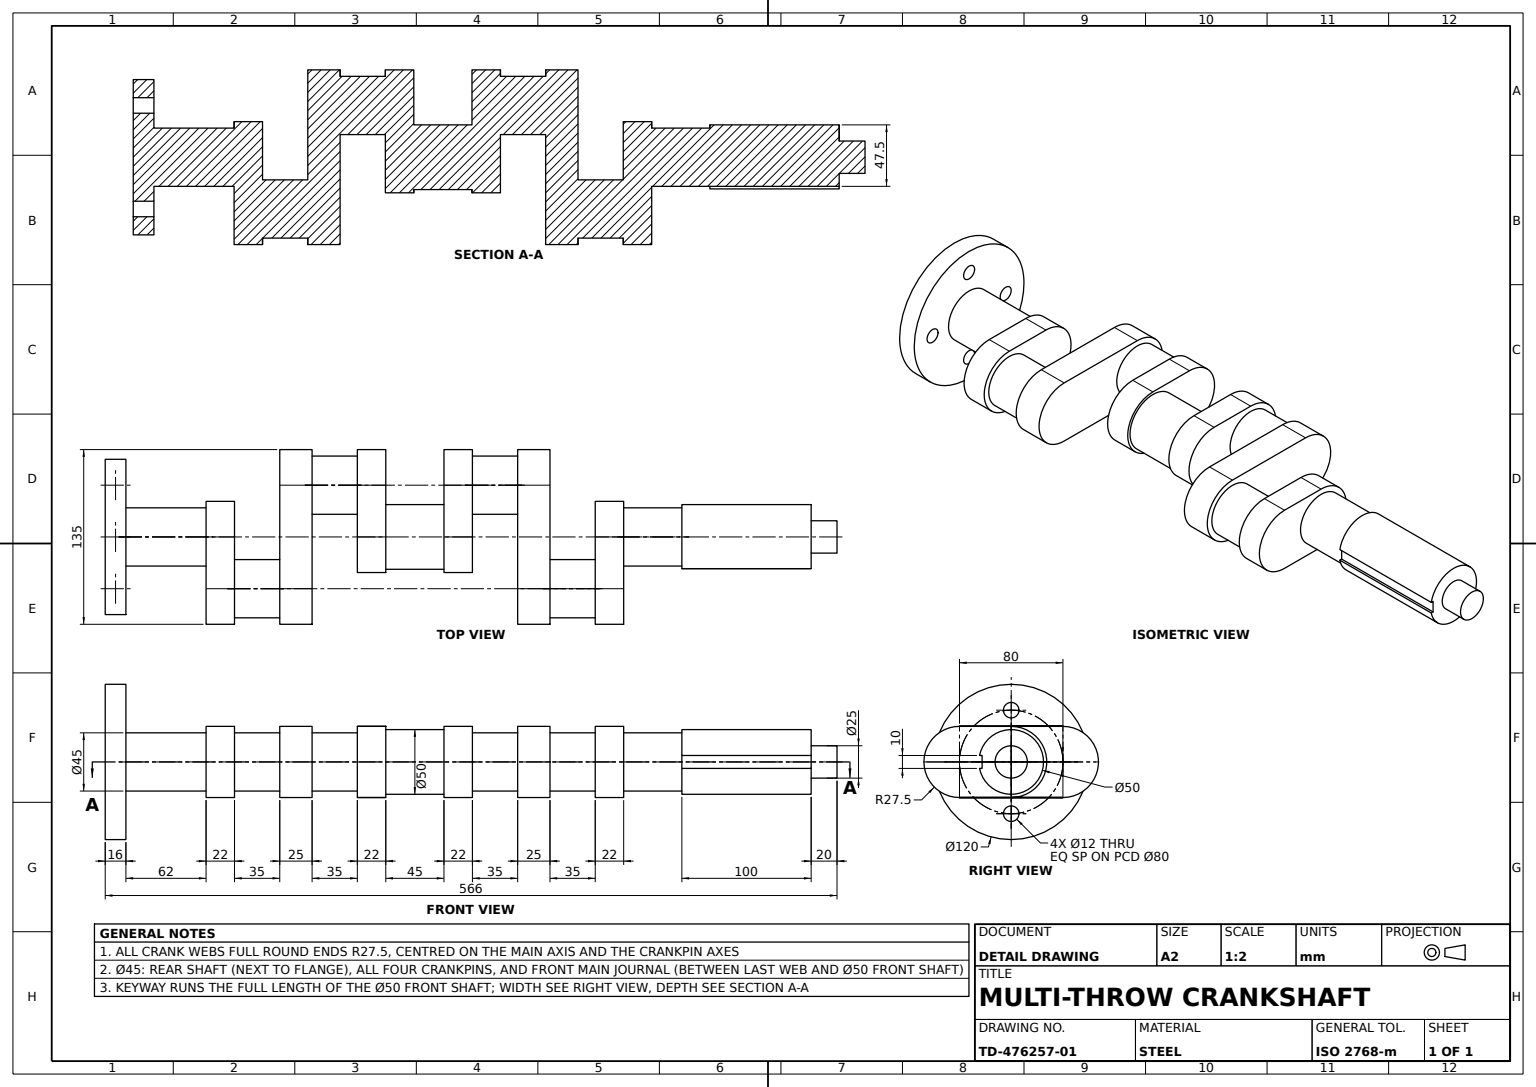
solid
v1 (262,-27.5,0)
v2 (262,-27.5,-40)
e1 v1 v2 LINE
v3 (262,0,27.5)
e2 v3 v1 CIRCLE(AX(P(262,0,0),D(1,0,0),D(0,0,-1)),27.5)
v4 (262,27.5,0)
e3 v4 v3 CIRCLE(AX(P(262,0,0),D(1,0,0),D(0,0,-1)),27.5)
v5 (262,27.5,-40)
e4 v5 v4 LINE
e5 v2 v5 CIRCLE(AX(P(262,0,-40),D(1,0,0),D(0,0,-1)),27.5)
v6 (262,0,25)
v7 (262,0,-25)
e6 v6 v7 CIRCLE(AX(P(262,0,0),D(1,0,0),D(0,0,-1)),25)
e7 v7 v6 CIRCLE(AX(P(262,0,0),D(1,0,0),D(0,0,-1)),25)
face PLANE(AX(P(262,0,0),D(1,0,0),D(0,0,-1))) rev [-e1 -e2 -e3 -e4 -e5] [e6 e7]
v8 (78,0,-22.5)
v9 (78,0,22.5)
e8 v8 v9 CIRCLE(AX(P(78,0,0),D(-1,0,0),D(0,0,1)),22.5)
e9 v9 v8 CIRCLE(AX(P(78,0,0),D(-1,0,0),D(0,0,1)),22.5)
v10 (78,0,67.5)
v11 (78,-27.5,40)
e10 v10 v11 CIRCLE(AX(P(78,0,40),D(1,0,0),D(0,0,-1)),27.5)
v12 (78,27.5,40)
e11 v12 v10 CIRCLE(AX(P(78,0,40),D(1,0,0),D(0,0,-1)),27.5)
v13 (78,27.5,0)
e12 v13 v12 LINE
v14 (78,-27.5,0)
e13 v14 v13 CIRCLE(AX(P(78,0,0),D(1,0,0),D(0,0,-1)),27.5)
e14 v11 v14 LINE
face PLANE(AX(P(78,0,0),D(1,0,0),D(0,0,-1))) rev [-e8 -e9] [-e10 -e11 -e12 -e13 -e14]
v15 (16,-40,6)
v16 (0,-40,6)
e15 v15 v16 LINE
v17 (16,-40,-6)
e16 v17 v15 CIRCLE(AX(P(16,-40,0),D(-1,0,0),D(0,0,1)),6)
v18 (0,-40,-6)
e17 v17 v18 LINE
e18 v18 v16 CIRCLE(AX(P(0,-40,0),D(-1,0,0),D(0,0,1)),6)
face CYL(AX(P(20,-40,0),D(-1,0,0),D(0,0,1)),6) rev [-e15 -e16 e17 e18]
v19 (160,-27.5,-40)
v20 (160,27.5,-40)
e19 v19 v20 CIRCLE(AX(P(160,0,-40),D(1,0,0),D(0,0,-1)),27.5)
v21 (160,27.5,40)
e20 v20 v21 LINE
v22 (160,0,67.5)
e21 v21 v22 CIRCLE(AX(P(160,0,40),D(1,0,0),D(0,0,-1)),27.5)
v23 (160,-27.5,40)
e22 v22 v23 CIRCLE(AX(P(160,0,40),D(1,0,0),D(0,0,-1)),27.5)
e23 v23 v19 LINE
v24 (160,0,-62.5)
v25 (160,0,-17.5)
e24 v24 v25 CIRCLE(AX(P(160,0,-40),D(1,0,0),D(0,0,-1)),22.5)
e25 v25 v24 CIRCLE(AX(P(160,0,-40),D(1,0,0),D(0,0,-1)),22.5)
face PLANE(AX(P(160,0,40),D(1,0,0),D(0,0,-1))) [e19 e20 e21 e22 e23] [-e24 -e25]
v26 (284,27.5,-40)
e26 v26 v5 LINE
v27 (284,27.5,0)
e27 v27 v4 LINE
e28 v26 v27 LINE
face PLANE(AX(P(284,27.5,0),D(0,-1,0),D(0,0,-1))) rev [e26 e4 -e27 -e28]
v28 (319,0,-62.5)
v29 (319,0,-17.5)
e29 v28 v29 CIRCLE(AX(P(319,0,-40),D(1,0,0),D(0,0,-1)),22.5)
e30 v29 v28 CIRCLE(AX(P(319,0,-40),D(1,0,0),D(0,0,-1)),22.5)
v30 (319,27.5,40)
v31 (319,0,67.5)
e31 v30 v31 CIRCLE(AX(P(319,0,40),D(1,0,0),D(0,0,-1)),27.5)
v32 (319,27.5,-40)
e32 v32 v30 LINE
v33 (319,-27.5,-40)
e33 v33 v32 CIRCLE(AX(P(319,0,-40),D(1,0,0),D(0,0,-1)),27.5)
v34 (319,-27.5,40)
e34 v34 v33 LINE
e35 v31 v34 CIRCLE(AX(P(319,0,40),D(1,0,0),D(0,0,-1)),27.5)
face PLANE(AX(P(319,0,-40),D(1,0,0),D(0,0,-1))) rev [e29 e30] [-e31 -e32 -e33 -e34 -e35]
v35 (217,27.5,-40)
v36 (217,27.5,0)
e36 v35 v36 LINE
v37 (217,0,27.5)
e37 v36 v37 CIRCLE(AX(P(217,0,0),D(1,0,0),D(0,0,-1)),27.5)
v38 (217,-27.5,0)
e38 v37 v38 CIRCLE(AX(P(217,0,0),D(1,0,0),D(0,0,-1)),27.5)
v39 (217,-27.5,-40)
e39 v38 v39 LINE
e40 v39 v35 CIRCLE(AX(P(217,0,-40),D(1,0,0),D(0,0,-1)),27.5)
v40 (217,0,25)
v41 (217,0,-25)
e41 v40 v41 CIRCLE(AX(P(217,0,0),D(1,0,0),D(0,0,-1)),25)
e42 v41 v40 CIRCLE(AX(P(217,0,0),D(1,0,0),D(0,0,-1)),25)
face PLANE(AX(P(217,0,-40),D(1,0,0),D(0,0,-1))) [e36 e37 e38 e39 e40] [-e41 -e42]
v42 (401,27.5,40)
v43 (401,0,67.5)
e43 v42 v43 CIRCLE(AX(P(401,0,40),D(1,0,0),D(0,0,-1)),27.5)
v44 (379,27.5,40)
e44 v42 v44 LINE
v45 (379,0,67.5)
e45 v44 v45 CIRCLE(AX(P(379,0,40),D(1,0,0),D(0,0,-1)),27.5)
e46 v43 v45 LINE
face CYL(AX(P(401,0,40),D(-1,0,0),D(0,0,1)),27.5) [-e43 e44 e45 -e46]
v46 (0,0,-34)
v47 (0,0,-46)
e47 v46 v47 CIRCLE(AX(P(0,0,-40),D(-1,0,0),D(0,0,1)),6)
v48 (16,0,-46)
e48 v48 v47 LINE
v49 (16,0,-34)
e49 v49 v48 CIRCLE(AX(P(16,0,-40),D(-1,0,0),D(0,0,1)),6)
e50 v49 v46 LINE
face CYL(AX(P(20,0,-40),D(-1,0,0),D(0,0,1)),6) rev [e47 -e48 -e49 e50]
v50 (446,5,22.5)
v51 (546,5,22.5)
e51 v50 v51 LINE
v52 (446,0,22.5)
e52 v52 v50 LINE
v53 (446,-5,22.5)
e53 v53 v52 LINE
v54 (546,-5,22.5)
e54 v53 v54 LINE
e55 v54 v51 LINE
face PLANE(AX(P(436,5,22.5),D(0,0,-1),D(-1,0,0))) rev [-e51 -e52 -e53 e54 e55]
v55 (566,0,12.5)
v56 (546,0,12.5)
e56 v55 v56 LINE
v57 (566,0,-12.5)
e57 v57 v55 CIRCLE(AX(P(566,0,0),D(1,0,0),D(0,0,-1)),12.5)
v58 (546,0,-12.5)
e58 v57 v58 LINE
e59 v58 v56 CIRCLE(AX(P(546,0,0),D(1,0,0),D(0,0,-1)),12.5)
face CYL(AX(P(566,0,0),D(-1,0,0),D(0,0,1)),12.5) [-e56 -e57 e58 e59]
e60 v15 v17 CIRCLE(AX(P(16,-40,0),D(-1,0,0),D(0,0,1)),6)
e61 v16 v18 CIRCLE(AX(P(0,-40,0),D(-1,0,0),D(0,0,1)),6)
face CYL(AX(P(20,-40,0),D(-1,0,0),D(0,0,1)),6) rev [-e60 e15 e61 -e17]
v59 (401,-27.5,0)
v60 (401,27.5,0)
e62 v59 v60 CIRCLE(AX(P(401,0,0),D(1,0,0),D(0,0,-1)),27.5)
e63 v60 v42 LINE
v61 (401,-27.5,40)
e64 v43 v61 CIRCLE(AX(P(401,0,40),D(1,0,0),D(0,0,-1)),27.5)
e65 v61 v59 LINE
v62 (401,0,22.5)
v63 (401,0,-22.5)
e66 v62 v63 CIRCLE(AX(P(401,0,0),D(1,0,0),D(0,0,-1)),22.5)
e67 v63 v62 CIRCLE(AX(P(401,0,0),D(1,0,0),D(0,0,-1)),22.5)
face PLANE(AX(P(401,0,40),D(1,0,0),D(0,0,-1))) [e62 e63 e43 e64 e65] [-e66 -e67]
v64 (446,5,24.494897)
v65 (546,5,24.494897)
e68 v64 v65 LINE
e69 v50 v64 LINE
e70 v51 v65 LINE
face PLANE(AX(P(436,5,27.5),D(0,1,0),D(0,0,1))) rev [-e68 -e69 e51 e70]
v66 (284,0,-17.5)
e71 v29 v66 LINE
v67 (284,0,-62.5)
e72 v66 v67 CIRCLE(AX(P(284,0,-40),D(1,0,0),D(0,0,-1)),22.5)
e73 v28 v67 LINE
face CYL(AX(P(319,0,-40),D(-1,0,0),D(0,0,1)),22.5) [e71 e72 -e73 -e30]
v68 (344,0,17.5)
v69 (344,0,62.5)
e74 v68 v69 CIRCLE(AX(P(344,0,40),D(1,0,0),D(0,0,-1)),22.5)
v70 (379,0,62.5)
e75 v70 v69 LINE
v71 (379,0,17.5)
e76 v71 v70 CIRCLE(AX(P(379,0,40),D(1,0,0),D(0,0,-1)),22.5)
e77 v71 v68 LINE
face CYL(AX(P(379,0,40),D(-1,0,0),D(0,0,1)),22.5) [e74 -e75 -e76 e77]
v72 (195,-27.5,0)
v73 (195,-27.5,-40)
e78 v72 v73 LINE
v74 (195,0,27.5)
e79 v74 v72 CIRCLE(AX(P(195,0,0),D(1,0,0),D(0,0,-1)),27.5)
v75 (195,27.5,0)
e80 v75 v74 CIRCLE(AX(P(195,0,0),D(1,0,0),D(0,0,-1)),27.5)
v76 (195,27.5,-40)
e81 v76 v75 LINE
e82 v73 v76 CIRCLE(AX(P(195,0,-40),D(1,0,0),D(0,0,-1)),27.5)
v77 (195,0,-62.5)
v78 (195,0,-17.5)
e83 v77 v78 CIRCLE(AX(P(195,0,-40),D(1,0,0),D(0,0,-1)),22.5)
e84 v78 v77 CIRCLE(AX(P(195,0,-40),D(1,0,0),D(0,0,-1)),22.5)
face PLANE(AX(P(195,0,-40),D(1,0,0),D(0,0,-1))) rev [-e78 -e79 -e80 -e81 -e82] [e83 e84]
v79 (135,0,62.5)
v80 (135,0,17.5)
e85 v79 v80 CIRCLE(AX(P(135,0,40),D(1,0,0),D(0,0,-1)),22.5)
e86 v80 v79 CIRCLE(AX(P(135,0,40),D(1,0,0),D(0,0,-1)),22.5)
v81 (135,-27.5,-40)
v82 (135,27.5,-40)
e87 v81 v82 CIRCLE(AX(P(135,0,-40),D(1,0,0),D(0,0,-1)),27.5)
v83 (135,-27.5,40)
e88 v83 v81 LINE
v84 (135,0,67.5)
e89 v84 v83 CIRCLE(AX(P(135,0,40),D(1,0,0),D(0,0,-1)),27.5)
v85 (135,27.5,40)
e90 v85 v84 CIRCLE(AX(P(135,0,40),D(1,0,0),D(0,0,-1)),27.5)
e91 v82 v85 LINE
face PLANE(AX(P(135,0,40),D(1,0,0),D(0,0,-1))) rev [e85 e86] [-e87 -e88 -e89 -e90 -e91]
v86 (16,0,-22.5)
e92 v8 v86 LINE
v87 (16,0,22.5)
e93 v87 v86 CIRCLE(AX(P(16,0,0),D(-1,0,0),D(0,0,1)),22.5)
e94 v9 v87 LINE
face CYL(AX(P(-89.08642,0,0),D(-1,0,0),D(0,0,1)),22.5) [e9 e92 -e93 -e94]
e95 v19 v81 LINE
e96 v20 v82 LINE
face CYL(AX(P(160,0,-40),D(-1,0,0),D(0,0,1)),27.5) [-e19 e95 e87 -e96]
v88 (16,40,6)
v89 (0,40,6)
e97 v88 v89 LINE
v90 (0,40,-6)
e98 v89 v90 CIRCLE(AX(P(0,40,0),D(-1,0,0),D(0,0,1)),6)
v91 (16,40,-6)
e99 v91 v90 LINE
e100 v88 v91 CIRCLE(AX(P(16,40,0),D(-1,0,0),D(0,0,1)),6)
face CYL(AX(P(20,40,0),D(-1,0,0),D(0,0,1)),6) rev [e97 e98 -e99 -e100]
v92 (379,-27.5,40)
e101 v45 v92 CIRCLE(AX(P(379,0,40),D(1,0,0),D(0,0,-1)),27.5)
e102 v61 v92 LINE
face CYL(AX(P(401,0,40),D(-1,0,0),D(0,0,1)),27.5) [-e64 e46 e101 -e102]
v93 (100,-27.5,0)
e103 v93 v14 LINE
v94 (100,27.5,0)
e104 v94 v13 LINE
e105 v93 v94 CIRCLE(AX(P(100,0,0),D(1,0,0),D(0,0,-1)),27.5)
face CYL(AX(P(100,0,0),D(-1,0,0),D(0,0,1)),27.5) [e103 e13 -e104 -e105]
v95 (446,0,-22.5)
e106 v95 v63 LINE
e107 v52 v95 CIRCLE(AX(P(446,0,0),D(1,0,0),D(0,0,-1)),22.5)
e108 v52 v62 LINE
face CYL(AX(P(446,0,0),D(-1,0,0),D(0,0,1)),22.5) [-e106 -e107 e108 e66]
e109 v35 v76 LINE
e110 v36 v75 LINE
face PLANE(AX(P(217,27.5,-40),D(0,-1,0),D(0,0,-1))) rev [e109 e81 -e110 -e36]
e111 v48 v49 CIRCLE(AX(P(16,0,-40),D(-1,0,0),D(0,0,1)),6)
e112 v47 v46 CIRCLE(AX(P(0,0,-40),D(-1,0,0),D(0,0,1)),6)
face CYL(AX(P(20,0,-40),D(-1,0,0),D(0,0,1)),6) rev [-e50 -e111 e48 e112]
v96 (284,0,27.5)
e113 v96 v3 LINE
e114 v27 v96 CIRCLE(AX(P(284,0,0),D(1,0,0),D(0,0,-1)),27.5)
face CYL(AX(P(284,0,0),D(-1,0,0),D(0,0,1)),27.5) [-e113 -e114 e27 e3]
v97 (379,27.5,0)
e115 v60 v97 LINE
e116 v97 v44 LINE
face PLANE(AX(P(401,27.5,40),D(0,-1,0),D(0,0,-1))) rev [-e44 -e63 e115 e116]
e117 v39 v73 LINE
face CYL(AX(P(217,0,-40),D(-1,0,0),D(0,0,1)),27.5) [-e40 e117 e82 -e109]
v98 (344,27.5,40)
e118 v98 v30 LINE
v99 (344,0,67.5)
e119 v99 v31 LINE
e120 v98 v99 CIRCLE(AX(P(344,0,40),D(1,0,0),D(0,0,-1)),27.5)
face CYL(AX(P(344,0,40),D(-1,0,0),D(0,0,1)),27.5) [e118 e31 -e119 -e120]
e121 v77 v24 LINE
e122 v78 v25 LINE
face CYL(AX(P(195,0,-40),D(-1,0,0),D(0,0,1)),22.5) [-e83 e121 e24 -e122]
v100 (100,27.5,40)
e123 v100 v12 LINE
e124 v94 v100 LINE
face PLANE(AX(P(100,27.5,0),D(0,-1,0),D(0,0,-1))) rev [e12 -e123 -e124 e104]
e125 v86 v87 CIRCLE(AX(P(16,0,0),D(-1,0,0),D(0,0,1)),22.5)
face CYL(AX(P(-89.08642,0,0),D(-1,0,0),D(0,0,1)),22.5) [-e125 -e92 e8 e94]
v101 (100,0,67.5)
v102 (100,-27.5,40)
e126 v101 v102 CIRCLE(AX(P(100,0,40),D(1,0,0),D(0,0,-1)),27.5)
e127 v101 v10 LINE
e128 v102 v11 LINE
face CYL(AX(P(100,0,40),D(-1,0,0),D(0,0,1)),27.5) [-e126 e127 e10 -e128]
v103 (284,-27.5,-40)
e129 v103 v26 CIRCLE(AX(P(284,0,-40),D(1,0,0),D(0,0,-1)),27.5)
e130 v103 v2 LINE
face CYL(AX(P(284,0,-40),D(-1,0,0),D(0,0,1)),27.5) [-e129 e130 e5 -e26]
v104 (0,0,34)
v105 (0,0,46)
e131 v104 v105 CIRCLE(AX(P(0,0,40),D(-1,0,0),D(0,0,1)),6)
v106 (16,0,46)
e132 v106 v105 LINE
v107 (16,0,34)
e133 v107 v106 CIRCLE(AX(P(16,0,40),D(-1,0,0),D(0,0,1)),6)
e134 v107 v104 LINE
face CYL(AX(P(20,0,40),D(-1,0,0),D(0,0,1)),6) rev [e131 -e132 -e133 e134]
e135 v100 v101 CIRCLE(AX(P(100,0,40),D(1,0,0),D(0,0,-1)),27.5)
face CYL(AX(P(100,0,40),D(-1,0,0),D(0,0,1)),27.5) [e123 e11 -e127 -e135]
v108 (546,-5,24.494897)
e136 v108 v54 LINE
v109 (446,-5,24.494897)
e137 v109 v53 LINE
e138 v108 v109 LINE
face PLANE(AX(P(436,-5,27.5),D(0,-1,0),D(0,0,-1))) rev [e136 -e54 -e137 -e138]
v110 (379,-27.5,0)
e139 v92 v110 LINE
e140 v59 v110 LINE
face PLANE(AX(P(401,-27.5,40),D(0,1,0),D(0,0,1))) rev [e139 -e140 -e65 e102]
e141 v38 v72 LINE
face PLANE(AX(P(217,-27.5,-40),D(0,1,0),D(0,0,1))) rev [-e117 -e39 e141 e78]
e142 v95 v52 CIRCLE(AX(P(446,0,0),D(1,0,0),D(0,0,-1)),22.5)
face CYL(AX(P(446,0,0),D(-1,0,0),D(0,0,1)),22.5) [-e142 e106 e67 -e108]
e143 v69 v68 CIRCLE(AX(P(344,0,40),D(1,0,0),D(0,0,-1)),22.5)
v111 (344,-27.5,40)
e144 v99 v111 CIRCLE(AX(P(344,0,40),D(1,0,0),D(0,0,-1)),27.5)
v112 (344,-27.5,-40)
e145 v111 v112 LINE
v113 (344,27.5,-40)
e146 v112 v113 CIRCLE(AX(P(344,0,-40),D(1,0,0),D(0,0,-1)),27.5)
e147 v113 v98 LINE
face PLANE(AX(P(344,0,-40),D(1,0,0),D(0,0,-1))) [-e143 -e74] [e144 e145 e146 e147 e120]
e148 v113 v32 LINE
face PLANE(AX(P(344,27.5,-40),D(0,-1,0),D(0,0,-1))) rev [e148 e32 -e118 -e147]
e149 v105 v104 CIRCLE(AX(P(0,0,40),D(-1,0,0),D(0,0,1)),6)
e150 v106 v107 CIRCLE(AX(P(16,0,40),D(-1,0,0),D(0,0,1)),6)
face CYL(AX(P(20,0,40),D(-1,0,0),D(0,0,1)),6) rev [e132 e149 -e134 -e150]
e151 v70 v71 CIRCLE(AX(P(379,0,40),D(1,0,0),D(0,0,-1)),22.5)
face CYL(AX(P(379,0,40),D(-1,0,0),D(0,0,1)),22.5) [-e151 e75 e143 -e77]
e152 v23 v83 LINE
face PLANE(AX(P(160,-27.5,40),D(0,1,0),D(0,0,1))) rev [-e23 e152 e88 -e95]
e153 v22 v84 LINE
face CYL(AX(P(160,0,40),D(-1,0,0),D(0,0,1)),27.5) [-e152 -e22 e153 e89]
e154 v110 v97 CIRCLE(AX(P(379,0,0),D(1,0,0),D(0,0,-1)),27.5)
face PLANE(AX(P(379,0,40),D(1,0,0),D(0,0,-1))) rev [e151 e76] [-e154 -e139 -e101 -e45 -e116]
e155 v55 v57 CIRCLE(AX(P(566,0,0),D(1,0,0),D(0,0,-1)),12.5)
face PLANE(AX(P(566,0,0),D(1,0,0),D(0,0,-1))) [e57 e155]
e156 v90 v89 CIRCLE(AX(P(0,40,0),D(-1,0,0),D(0,0,1)),6)
e157 v91 v88 CIRCLE(AX(P(16,40,0),D(-1,0,0),D(0,0,1)),6)
face CYL(AX(P(20,40,0),D(-1,0,0),D(0,0,1)),6) rev [e99 e156 -e97 -e157]
v114 (16,0,-60)
v115 (0,0,-60)
e158 v114 v115 LINE
v116 (0,0,60)
e159 v116 v115 CIRCLE(AX(P(0,0,0),D(-1,0,0),D(0,0,1)),60)
v117 (16,0,60)
e160 v117 v116 LINE
e161 v117 v114 CIRCLE(AX(P(16,0,0),D(-1,0,0),D(0,0,1)),60)
face CYL(AX(P(-89.08642,0,0),D(-1,0,0),D(0,0,1)),60) [e158 -e159 -e160 e161]
v118 (284,-27.5,0)
e162 v118 v1 LINE
e163 v96 v118 CIRCLE(AX(P(284,0,0),D(1,0,0),D(0,0,-1)),27.5)
face CYL(AX(P(284,0,0),D(-1,0,0),D(0,0,1)),27.5) [-e162 -e163 e113 e2]
e164 v114 v117 CIRCLE(AX(P(16,0,0),D(-1,0,0),D(0,0,1)),60)
face PLANE(AX(P(16,60,0),D(-1,0,0),D(0,0,1))) rev [e93 e125] [-e161 -e164] [e133 e150] [e49 e111] [e60 e16] [e157 e100]
e165 v21 v85 LINE
face CYL(AX(P(160,0,40),D(-1,0,0),D(0,0,1)),27.5) [-e153 -e21 e165 e90]
e166 v115 v116 CIRCLE(AX(P(0,0,0),D(-1,0,0),D(0,0,1)),60)
face PLANE(AX(P(0,0,0),D(1,0,0),D(0,0,-1))) rev [-e61 -e18] [-e156 -e98] [-e131 -e149] [e159 e166] [-e47 -e112]
v119 (100,0,17.5)
e167 v80 v119 LINE
v120 (100,0,62.5)
e168 v119 v120 CIRCLE(AX(P(100,0,40),D(1,0,0),D(0,0,-1)),22.5)
e169 v79 v120 LINE
face CYL(AX(P(135,0,40),D(-1,0,0),D(0,0,1)),22.5) [-e86 e167 e168 -e169]
face CYL(AX(P(195,0,-40),D(-1,0,0),D(0,0,1)),22.5) [-e121 -e84 e122 e25]
e170 v120 v119 CIRCLE(AX(P(100,0,40),D(1,0,0),D(0,0,-1)),22.5)
face CYL(AX(P(135,0,40),D(-1,0,0),D(0,0,1)),22.5) [-e85 e169 e170 -e167]
e171 v6 v40 LINE
e172 v7 v41 LINE
face CYL(AX(P(262,0,0),D(-1,0,0),D(0,0,1)),25) [-e171 -e7 e172 e42]
e173 v111 v34 LINE
face CYL(AX(P(344,0,40),D(-1,0,0),D(0,0,1)),27.5) [-e144 e119 e35 -e173]
e174 v37 v74 LINE
face CYL(AX(P(217,0,0),D(-1,0,0),D(0,0,1)),27.5) [e79 -e141 -e38 e174]
e175 v102 v93 LINE
face PLANE(AX(P(100,-27.5,0),D(0,1,0),D(0,0,1))) rev [e128 e14 -e103 -e175]
face CYL(AX(P(401,0,0),D(-1,0,0),D(0,0,1)),27.5) [e154 -e115 -e62 e140]
e176 v56 v58 CIRCLE(AX(P(546,0,0),D(1,0,0),D(0,0,-1)),12.5)
face CYL(AX(P(566,0,0),D(-1,0,0),D(0,0,1)),12.5) [e176 -e58 -e155 e56]
e177 v67 v66 CIRCLE(AX(P(284,0,-40),D(1,0,0),D(0,0,-1)),22.5)
face CYL(AX(P(319,0,-40),D(-1,0,0),D(0,0,1)),22.5) [-e29 e73 e177 -e71]
e178 v109 v64 CIRCLE(AX(P(446,0,0),D(1,0,0),D(0,0,-1)),25)
face PLANE(AX(P(446,0,0),D(1,0,0),D(0,0,-1))) rev [-e178 e137 e53 e107 e142 e52 e69]
e179 v118 v103 LINE
face PLANE(AX(P(284,-27.5,0),D(0,1,0),D(0,0,1))) rev [e1 -e130 -e179 e162]
face CYL(AX(P(217,0,0),D(-1,0,0),D(0,0,1)),27.5) [e80 -e174 -e37 e110]
face PLANE(AX(P(100,0,0),D(1,0,0),D(0,0,-1))) [e126 e175 e105 e124 e135] [-e168 -e170]
face PLANE(AX(P(160,27.5,40),D(0,-1,0),D(0,0,-1))) rev [-e165 -e20 e96 e91]
face CYL(AX(P(262,0,0),D(-1,0,0),D(0,0,1)),25) [e41 -e172 -e6 e171]
face CYL(AX(P(-89.08642,0,0),D(-1,0,0),D(0,0,1)),60) [e160 -e166 -e158 e164]
face PLANE(AX(P(284,0,0),D(1,0,0),D(0,0,-1))) [-e72 -e177] [e179 e129 e28 e114 e163]
e180 v108 v65 CIRCLE(AX(P(546,0,0),D(1,0,0),D(0,0,-1)),25)
face PLANE(AX(P(546,0,0),D(1,0,0),D(0,0,-1))) [-e70 -e55 -e136 e180] [-e176 -e59]
face CYL(AX(P(546,0,0),D(-1,0,0),D(0,0,1)),25) [e178 e68 -e180 e138]
e181 v112 v33 LINE
face CYL(AX(P(344,0,-40),D(-1,0,0),D(0,0,1)),27.5) [e181 e33 -e148 -e146]
face PLANE(AX(P(344,-27.5,-40),D(0,1,0),D(0,0,1))) rev [-e181 -e145 e173 e34]
